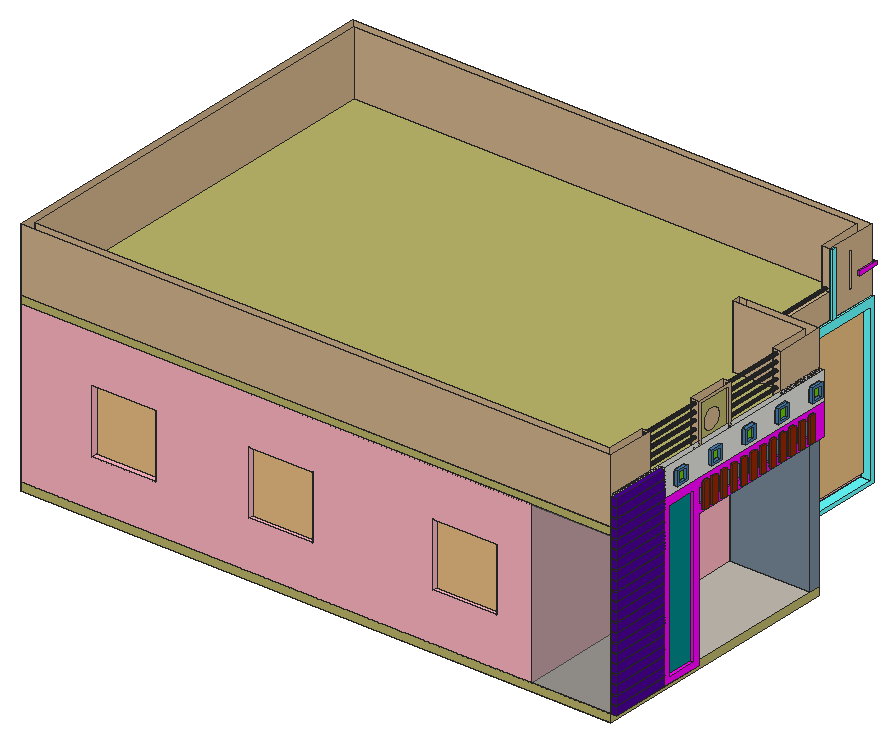
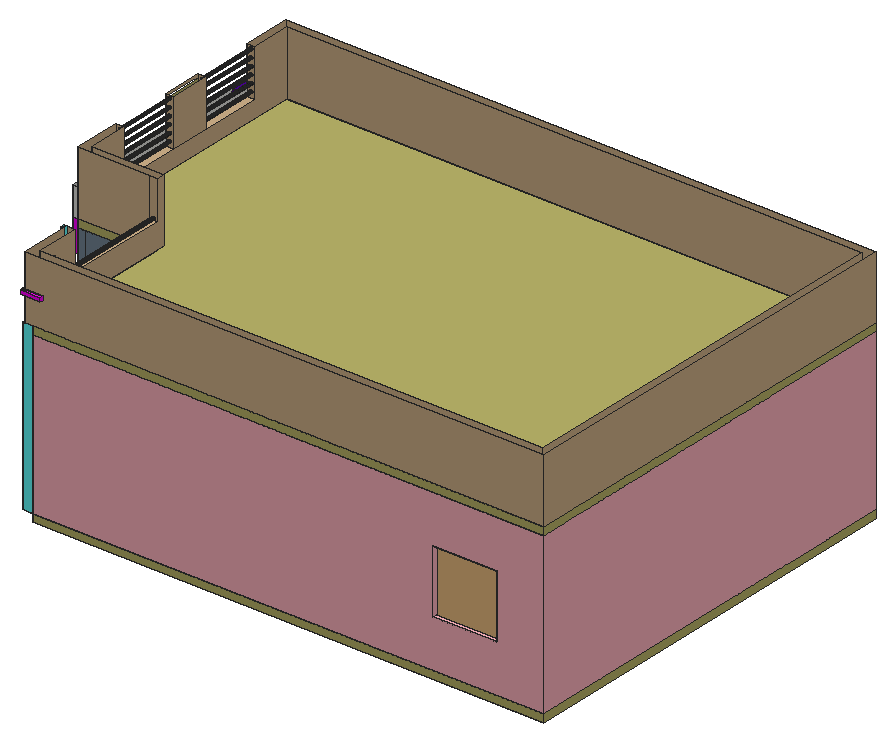
# SketchUp Ruby script. Lengths in inches.
U = 1.inch
M = Sketchup.active_model
def pt(a) = Geom::Point3d.new(a.map { |v| v * U })
def face(e, loops, mat)
  f = e.add_face(loops[0].map { |a| pt(a) })
  loops[1..].each { |l| e.add_face(l.map { |a| pt(a) }).erase! }
  f.material = f.back_material = mat if mat
  f
end
# faces: each face lists its corners as indices into pts; further lists are holes
def faces(e, pts, list, mat = nil) = list.each { |f| face(e, (f[0].is_a?(Array) ? f : [f]).map { |l| l.map { |i| pts[i] } }, mat) }
# xy, xz, yz: faces in a plane at the given z, y or x. An outline is a flat list of corners, or four numbers for a rectangle; further outlines are holes
def ring(l) = l.size == 4 ? [[l[0], l[1]], [l[2], l[1]], [l[2], l[3]], [l[0], l[3]]] : l.each_slice(2).to_a
def flat(e, list, mat, &to3) = list.each { |f| face(e, (f[0].is_a?(Array) ? f : [f]).map { |l| ring(l).map { |u, v| to3.(u, v) } }, mat) }
def xy(e, z, list, mat = nil) = flat(e, list, mat) { |x, y| [x, y, z] }
def xz(e, y, list, mat = nil) = flat(e, list, mat) { |x, z| [x, y, z] }
def yz(e, x, list, mat = nil) = flat(e, list, mat) { |y, z| [x, y, z] }
def lines(e, pts, list) = list.each { |a, b| e.add_line(pt(pts[a]), pt(pts[b])) }
# prism: a flat outline (further loops are holes) pulled along v
def prism(e, loops, v, mat = nil)
  f = face(e, loops, mat); d = Geom::Vector3d.new(v.map { |x| x * U })
  f.pushpull(f.normal.samedirection?(d) ? d.length : -d.length)
end
def box(e, o, s, mat = nil) = prism(e, [[o, [o[0] + s[0], o[1], o[2]], [o[0] + s[0], o[1] + s[1], o[2]], [o[0], o[1] + s[1], o[2]]]], [0, 0, s[2]], mat)
def at(x, y, z, deg = 0) = Geom::Transformation.translation(pt([x, y, z])) * Geom::Transformation.rotation(ORIGIN, Z_AXIS, deg.degrees)
def axes(o, x, y, z) = Geom::Transformation.new([*x, 0, *y, 0, *z, 0, *pt(o).to_a, 1])
def part(name) = M.definitions.add(name)
# library, detail: a bought-in or finely detailed component or shape, given as its bounding box
def library(name, o, s) = part(name).tap { |d| box(d.entities, o, s) }
def detail(e, o, s) = box(e.add_group.entities, o, s)
def put(e, d, t, mat = nil) = e.add_instance(d, t).tap { |i| i.material = mat if mat }
def group(e, t, mat = nil) = e.add_group.tap { |g| g.transformation = t; g.material = mat if mat }.entities
root = M.entities
M.materials.add("[0003_DeepPink]").color = [255, 20, 147]
M.materials.add("[0005_LightPink]").color = [255, 182, 193]
M.materials.add("[0035_Tan]").color = [210, 180, 140]
M.materials.add("[0057_DarkKhaki]").color = [189, 183, 107]
M.materials.add("[0080_DarkCyan]").color = [0, 139, 139]
M.materials.add("[0100_SteelBlue]").color = [70, 130, 180]
M.materials.add("[0109_DarkSlateBlue]").color = [72, 61, 139]
M.materials.add("[0110_LightSlateGray]").color = [119, 136, 153]
M.materials.add("[0127_Magenta]").color = [255, 0, 255]
M.materials.add("[0136_Charcoal]").color = [35, 35, 35]
M.materials.add("[Color B07]").color = [153, 38, 0]
M.materials.add("[Color F06]").color = [102, 204, 0]
M.materials.add("[Color H03]").color = [101, 255, 255]
M.materials.add("[Color J07]").color = [76, 0, 153]
M.materials.add("[Field Rectangle Tile]").color = [196, 189, 179]
M.materials.add("[Translucent Glass Gray]").color = [128, 128, 128]
M.materials["[Translucent Glass Gray]"].alpha = 0.5
c1 = library("BED 3",[-244.73,-59.6875,196.6875],[91.01,69.4,39.64])
c2 = library("建立群組\#166",[-1.39,17.71,0],[5.33,43.31,86.61])
c3 = library("Группа\#16",[0,0,0],[5.38,37.87,81.85])
c4 = library("Component",[269.12,209.03,0],[24,4.72,84.37])
c5 = library("Group\#20",[0,0,6],[2,110.9,114])
c6 = library("mesh-166",[-1553.69,-2604.3125,-42.18],[1702.88,1401.6,88.28])
c7 = part("Group17")
put(c7.entities,c6,at(294.66,859.51,3.5))
c8 = library("mesh-158",[272.88,-1887.9,-41.96],[1017.57,1401.85,65.81])
c9 = part("Component\#4")
box(c9.entities,[2.75,0,0],[18.9375,4.3125,2],"[Color B07]")
c10 = part("Component\#3")
xy(c10.entities,0,[[0,0,3,9.4375]],"[0100_SteelBlue]")
xy(c10.entities,1.08,[[0,1.08,0.1875,8.36],[0.1875,1.08,3,8.36]],"[0100_SteelBlue]")
xy(c10.entities,9.29,[[0,1.08,0.1875,8.36],[0.1875,1.08,3,8.36]],"[0100_SteelBlue]")
xy(c10.entities,10.375,[[0,0,3,9.4375]],"[0100_SteelBlue]")
xz(c10.entities,0,[[0,0,3,10.375]],"[0100_SteelBlue]")
xz(c10.entities,1.08,[[0,1.08,0.1875,9.29],[0.1875,1.08,3,9.29]],"[0100_SteelBlue]")
xz(c10.entities,8.36,[[0,1.08,0.1875,9.29],[0.1875,1.08,3,9.29]],"[0100_SteelBlue]")
xz(c10.entities,9.4375,[[0,0,3,10.375]],"[0100_SteelBlue]")
yz(c10.entities,0,[[[0,0,9.4375,10.375],[1.08,1.08,8.36,9.29]]],"[0100_SteelBlue]")
yz(c10.entities,0.1875,[[1.08,1.08,8.36,9.29]],"[Color F06]")
yz(c10.entities,3,[[[0,0,9.4375,10.375],[1.08,1.08,8.36,9.29]]],"[0100_SteelBlue]")
c11 = part("Round post")
xy(c11.entities,0,[[1,0,0.74,0.03,0.5,0.13,0.29,0.29,0.13,0.5,0.03,0.74,0,1,0.03,1.26,0.13,1.5,0.29,1.71,0.5,1.87,0.74,1.97,1,2,1.26,1.97,1.5,1.87,1.71,1.71,1.87,1.5,1.97,1.26,2,1,1.97,0.74,1.87,0.5,1.71,0.29,1.5,0.13,1.26,0.03]],"[0035_Tan]")
xy(c11.entities,46.55,[[1,0,1.26,0.03,1.5,0.13,1.71,0.29,1.87,0.5,1.97,0.74,2,1,1.97,1.26,1.87,1.5,1.71,1.71,1.5,1.87,1.26,1.97,1,2,0.74,1.97,0.5,1.87,0.29,1.71,0.13,1.5,0.03,1.26,0,1,0.03,0.74,0.13,0.5,0.29,0.29,0.5,0.13,0.74,0.03]],"[0035_Tan]")
p = [[0.5,0.13,0],[0.74,0.03,0],[0.74,0.03,46.55],[0.5,0.13,46.55],[1,0,0],[1,0,46.55],
  [1.26,0.03,0],[1.26,0.03,46.55],[1.5,0.13,0],[1.5,0.13,46.55],[0.29,0.29,0],[0.29,0.29,46.55],
  [1.71,0.29,0],[1.71,0.29,46.55],[0.13,0.5,0],[0.13,0.5,46.55],[1.87,0.5,0],[1.87,0.5,46.55],
  [0.03,0.74,0],[0.03,0.74,46.55],[1.97,0.74,0],[1.97,0.74,46.55],[0,1,0],[0,1,46.55],
  [2,1,0],[2,1,46.55],[0.03,1.26,0],[0.03,1.26,46.55],[1.97,1.26,0],[1.97,1.26,46.55],
  [0.13,1.5,0],[0.13,1.5,46.55],[1.87,1.5,0],[1.87,1.5,46.55],[0.29,1.71,0],[0.29,1.71,46.55],
  [1.71,1.71,0],[1.71,1.71,46.55],[0.5,1.87,0],[0.5,1.87,46.55],[1.5,1.87,0],[1.5,1.87,46.55],
  [0.74,1.97,0],[0.74,1.97,46.55],[1.26,1.97,0],[1.26,1.97,46.55],[1,2,0],[1,2,46.55]]
faces(c11.entities,p,[[0,1,2,3],[1,4,5,2],[4,6,7,5],[6,8,9,7],[10,0,3,11],[8,12,13,9],[14,10,11,15],[12,16,17,13],
  [18,14,15,19],[16,20,21,17],[22,18,19,23],[20,24,25,21],[26,22,23,27],[24,28,29,25],[30,26,27,31],[28,32,33,29],
  [34,30,31,35],[32,36,37,33],[38,34,35,39],[36,40,41,37],[42,38,39,43],[40,44,45,41],[46,42,43,47],[44,46,47,45]],"[0136_Charcoal]")
c12 = part("Group\#26")
put(c12.entities,c11,axes([2,11.53,0],[-1,0,0],[0,1,0],[0,0,-1]))
put(c12.entities,c11,axes([2,17.29,0],[-1,0,0],[0,1,0],[0,0,-1]))
put(c12.entities,c11,axes([2,5.76,0],[-1,0,0],[0,1,0],[0,0,-1]))
put(c12.entities,c11,axes([2,23.05,0],[-1,0,0],[0,1,0],[0,0,-1]))
put(c12.entities,c11,axes([2,28.8125,0],[-1,0,0],[0,1,0],[0,0,-1]))
put(c12.entities,c11,axes([2,0,0],[-1,0,0],[0,1,0],[0,0,-1]))
c13 = part("Group\#24")
prism(c13.entities,[[[2.25,1.125,0],[2.21,0.83,0],[2.1,0.5625,0],[1.92,0.33,0],[1.6875,0.15,0],[1.42,0.04,0],[1.125,0,0],[0.83,0.04,0],[0.5625,0.15,0],[0.33,0.33,0],[0.15,0.5625,0],[0.04,0.83,0],[0,1.125,0],[0.04,1.42,0],[0.15,1.6875,0],[0.33,1.92,0],[0.5625,2.1,0],[0.83,2.21,0],[1.125,2.25,0],[1.42,2.21,0],[1.6875,2.1,0],[1.92,1.92,0],[2.1,1.6875,0],[2.21,1.42,0]]],[0,0,77.9])
c14 = part("Component\#2")
xy(c14.entities,-13,[[13.51,0,15.51,2.94]],"[0127_Magenta]")
xy(c14.entities,2,[[0,0,15.51,2.94]],"[0127_Magenta]")
xz(c14.entities,0,[[13.51,-13,15.51,0],[0,0,15.51,2]],"[0127_Magenta]")
xz(c14.entities,2.94,[[13.51,-13,15.51,2],[0,0,13.51,2]],"[0127_Magenta]")
yz(c14.entities,0,[[0,0,2.94,2]],"[0127_Magenta]")
yz(c14.entities,13.51,[[0,-13,2.94,2]],"[0127_Magenta]")
yz(c14.entities,15.51,[[0,-13,2.94,2]],"[0127_Magenta]")
xy(root,0,[[384,188.1,444,197.1]],"[0109_DarkSlateBlue]")
xy(root,0,[[444,2,448,79.01]],"[Color J07]")
xy(root,4,[[445,51.2,448,75.01]],"[0127_Magenta]")
xy(root,6,[[444,2,448,47.2]],"[Color J07]")
xy(root,7,[[444,2,448,47.2]])
xy(root,13,[[444,2,448,47.2]],"[Color J07]")
xy(root,14,[[444,2,448,47.2]])
xy(root,20,[[444,2,448,47.2]],"[Color J07]")
xy(root,21,[[444,2,448,47.2]])
xy(root,27,[[444,2,448,47.2]],"[Color J07]")
xy(root,28,[[444,2,448,47.2]])
xy(root,34,[[444,2,448,47.2]],"[Color J07]")
xy(root,35,[[444,2,448,47.2]],"[Color J07]")
xy(root,41,[[444,2,448,47.2]],"[Color J07]")
xy(root,42,[[444,2,448,47.2]],"[Color J07]")
xy(root,48,[[444,2,448,47.2]],"[Color J07]")
xy(root,49,[[444,2,448,47.2]],"[Color J07]")
xy(root,55,[[444,2,448,47.2]],"[Color J07]")
xy(root,56,[[444,2,448,47.2]],"[Color J07]")
xy(root,62,[[444,2,448,47.2]],"[Color J07]")
xy(root,63,[[444,2,448,47.2]],"[Color J07]")
xy(root,69,[[444,2,448,47.2]],"[Color J07]")
xy(root,70,[[444,2,448,47.2]],"[Color J07]")
xy(root,76,[[444,2,448,47.2]],"[Color J07]")
xy(root,77,[[444,2,448,47.2]],"[Color J07]")
xy(root,83,[[444,2,448,47.2]],"[Color J07]")
xy(root,84,[[444,2,448,47.2]],"[Color J07]")
xy(root,90,[[444,2,448,47.2]],"[Color J07]")
xy(root,91,[[444,2,448,47.2]],"[Color J07]")
xy(root,97,[[444,2,448,47.2]],"[Color J07]")
xy(root,98,[[444,2,448,47.2]],"[Color J07]")
xy(root,102,[[444,79.01,448,197.1]],"[0127_Magenta]")
xy(root,104,[[444,2,448,47.2]],"[Color J07]")
xy(root,105,[[444,2,448,47.2]],"[Color J07]")
xy(root,108,[[444,79.01,446,188.1],[446,79.01,448,188.1]],"[0127_Magenta]")
xy(root,111,[[444,2,448,47.2]],"[Color J07]")
xy(root,112,[[444,2,448,47.2]],"[Color J07]")
xy(root,118,[[444,2,448,47.2]],"[Color J07]")
xy(root,119,[[444,2,448,47.2]],"[Color J07]")
xy(root,119.875,[[445,51.2,448,75.01],[444,79.01,446,188.1],[446,79.01,448,188.1]],"[0127_Magenta]")
xy(root,120,[[384,188.1,444,197.1]],"[0109_DarkSlateBlue]")
xy(root,125,[[444,2,448,47.2]],"[Color J07]")
xy(root,126,[[[0,2,0,314,390,314,390,197.1,444,197.1,444,2],[6,8,438,8,438,191.1,384,191.1,384,308,6,308]]],"[0035_Tan]")
xy(root,126,[[444,2,448,47.2]],"[Color J07]")
xy(root,132,[[444,2,448,47.2]],"[Color J07]")
xy(root,133,[[444,2,448,47.2]],"[Color J07]")
xy(root,138.27,[[384,292.3,390,295.12]],"[0035_Tan]")
xy(root,138.5,[[438,38,444,84.55],[438,84.55,444,114.55],[438,114.55,444,161.1]],"[0035_Tan]")
xy(root,139,[[444,2,448,47.2]],"[Color J07]")
xy(root,140,[[444,2,448,47.2]],"[Color J07]")
xy(root,140.5,[[442,86.55,444,112.55]],"[0035_Tan]")
xy(root,145.18,[[384,197.1,390,275]],"[0035_Tan]")
xy(root,146,[[444,2,448,47.2]],"[Color J07]")
xz(root,2,[[0,126,444,174]],"[0035_Tan]")
xz(root,2,[[444,0,448,6],[444,7,448,13],[444,14,448,20],[444,21,448,27],[444,28,448,34],
  [444,35,448,41],[444,42,448,48],[444,49,448,55],[444,56,448,62],[444,63,448,69],
  [444,70,448,76],[444,77,448,83],[444,84,448,90],[444,91,448,97],[444,98,448,104],
  [444,105,448,111],[444,112,448,118],[444,119,448,125],[444,126,448,132],[444,133,448,139],
  [444,140,448,146]],"[Color J07]")
xz(root,2,[[384,0,444,120]],"[Translucent Glass Gray]")
xz(root,8,[[6,126,438,174]],"[0035_Tan]")
xz(root,38,[[438,138.5,444,174]],"[0035_Tan]")
xz(root,47.2,[[444,6,448,7],[444,13,448,14],[444,20,448,21],[444,27,448,28],[444,34,448,35],
  [444,41,448,42],[444,48,448,49],[444,55,448,56],[444,62,448,63],[444,69,448,70],
  [444,76,448,77],[444,83,448,84],[444,90,448,91],[444,97,448,98],[444,104,448,105],
  [444,111,448,112],[444,118,448,119],[444,125,448,126],[444,132,448,133],[444,139,448,140],
  [444,146,448,147]])
xz(root,51.2,[[445,4,448,119.875]],"[0127_Magenta]")
xz(root,75.01,[[445,4,448,119.875]],"[0127_Magenta]")
xz(root,79.01,[[444,0,448,102],[444,102,448,108],[444,108,446,119.875],[446,108,448,119.875]],"[0127_Magenta]")
xz(root,84.55,[[438,138.5,444,174]],"[0035_Tan]")
xz(root,86.55,[[442,140.5,444,172]],"[0035_Tan]")
xz(root,112.55,[[442,140.5,444,172]],"[0035_Tan]")
xz(root,114.55,[[438,138.5,444,174]],"[0035_Tan]")
xz(root,161.1,[[438,138.5,444,174]],"[0035_Tan]")
xz(root,188.1,[[384,0,444,120]],"[0110_LightSlateGray]")
xz(root,188.1,[[446,108,448,119.875]],"[0127_Magenta]")
xz(root,191.1,[[384,126,438,174]],"[0035_Tan]")
xz(root,197.1,[[444,126,448,147.28]])
xz(root,197.1,[[390,126,444,174],[384,145.18,390,174]],"[0035_Tan]")
xz(root,197.1,[[384,0,438,120],[438,0,444,120]],"[0110_LightSlateGray]")
xz(root,197.1,[[444,102,448,126]],"[0127_Magenta]")
xz(root,275,[[384,145.18,390,174]],"[0035_Tan]")
xz(root,292.3,[[384,138.27,390,165.21]],"[0035_Tan]")
xz(root,295.12,[[384,138.27,390,165.21]],"[0035_Tan]")
xz(root,308,[[6,126,384,174]],"[0035_Tan]")
xz(root,314,[[0,126,390,174]],"[0035_Tan]")
yz(root,0,[[2,126,314,174]],"[0035_Tan]")
yz(root,6,[[8,126,308,174]],"[0035_Tan]")
yz(root,384,[[[191.1,126,191.1,174,197.1,174,197.1,145.18,275,145.18,275,174,308,174,308,126],[292.3,138.27,295.12,165.21]]],"[0035_Tan]")
yz(root,384,[[188.1,0,197.1,120]],"[0109_DarkSlateBlue]")
yz(root,390,[[197.1,126,275,145.18],[[278,126,314,174],[292.3,138.27,295.12,165.21]]],"[0035_Tan]")
yz(root,438,[[8,126,8,174,38,174,38,138.5,161.1,138.5,161.1,174,191.1,174,191.1,126],[84.55,138.5,114.55,174]],"[0035_Tan]")
yz(root,442,[[[86.55,140.5,112.55,172],[98.5,147.98,98.02,148.01,97.54,148.07,97.0625,148.16,96.59,148.28,96.13,148.43,95.69,148.61,95.25,148.82,94.82,149.05,94.42,149.3125,94.03,149.6,93.65,149.91,93.3,150.24,92.97,150.59,92.66,150.96,92.38,151.35,92.12,151.76,91.89,152.1875,91.68,152.625,91.51,153.07,91.36,153.53,91.24,154,91.15,154.48,91.09,154.96,91.06,155.4375,91.06,155.92,91.09,156.41,91.15,156.88,91.24,157.36,91.36,157.83,91.51,158.29,91.69,158.74,91.9,159.17,92.13,159.6,92.39,160.01,92.67,160.4,92.98,160.77,93.3125,161.12,93.67,161.45,94.04,161.76,94.43,162.04,94.84,162.3,95.26,162.53,95.7,162.74,96.15,162.92,96.61,163.07,97.08,163.1875,97.55,163.28,98.03,163.34,98.52,163.37,99,163.37,99.48,163.33,99.96,163.27,100.4375,163.18,100.9,163.0625,101.36,162.91,101.8125,162.73,102.25,162.53,102.67,162.29,103.08,162.03,103.47,161.75,103.85,161.44,104.2,161.11,104.53,160.76,104.84,160.38,105.12,159.99,105.38,159.58,105.61,159.16,105.82,158.72,105.99,158.27,106.14,157.8125,106.26,157.34,106.35,156.87,106.41,156.39,106.44,155.91,106.44,155.42,106.41,154.94,106.35,154.46,106.26,153.99,106.14,153.52,105.99,153.06,105.81,152.61,105.6,152.17,105.37,151.75,105.11,151.34,104.83,150.95,104.52,150.58,104.1875,150.22,103.83,149.89,103.46,149.59,103.07,149.3,102.66,149.04,102.24,148.8125,101.8,148.61,101.35,148.43,100.89,148.28,100.42,148.16,99.95,148.07,99.47,148.01,98.98,147.98]]],"[0057_DarkKhaki]")
yz(root,444,[[2,0,2,6,47.2,6,47.2,7,2,7,2,13,47.2,13,47.2,14,2,14,2,20,47.2,20,47.2,21,2,21,2,27,47.2,27,47.2,28,2,28,2,34,47.2,34,47.2,35,2,35,2,41,47.2,41,47.2,42,2,42,2,48,47.2,48,47.2,49,2,49,2,55,47.2,55,47.2,56,2,56,2,62,47.2,62,47.2,63,2,63,2,69,47.2,69,47.2,70,2,70,2,76,47.2,76,47.2,77,2,77,2,83,47.2,83,47.2,84,2,84,2,90,47.2,90,47.2,91,2,91,2,97,47.2,97,47.2,98,2,98,2,104,47.2,104,47.2,105,2,105,2,111,47.2,111,47.2,112,2,112,2,118,47.2,118,47.2,119,2,119,2,125,47.2,125,47.2,126,2,126,2,132,47.2,132,47.2,133,2,133,2,139,47.2,139,47.2,140,2,140,2,146,47.2,146,47.2,147,2,147,2,147.28,197.1,147.28,197.1,120,188.1,120,188.1,119.875,79.01,119.875,79.01,0],[2,6,47.2,7],[2,13,47.2,14],[2,20,47.2,21],[2,27,47.2,28],
  [2,34,47.2,35],[2,41,47.2,42],[2,48,47.2,49],[2,55,47.2,56],[2,62,47.2,63],
  [2,69,47.2,70],[2,76,47.2,77],[2,83,47.2,84],[2,97,47.2,98],[2,104,47.2,105],
  [2,111,47.2,112],[2,118,47.2,119]])
yz(root,444,[[2,126,38,174],[38,126,161.1,138.5],[161.1,126,197.1,174],[[84.55,138.5,114.55,174],[86.55,140.5,112.55,172]]],"[0035_Tan]")
yz(root,444,[[188.1,102,197.1,120]],"[0109_DarkSlateBlue]")
yz(root,444,[[188.1,0,197.1,102]],"[0110_LightSlateGray]")
yz(root,444,[[79.01,102,188.1,108],[79.01,108,188.1,119.875]],"[0127_Magenta]")
yz(root,444,[[2,90,47.2,91]],"[Color J07]")
yz(root,445,[[51.2,4,75.01,119.875]],"[0080_DarkCyan]")
yz(root,446,[[79.01,108,188.1,119.875]],"[0110_LightSlateGray]")
yz(root,448,[[[47.2,0,79.01,0,79.01,102,197.1,102,197.1,126,47.2,126],[51.2,4,75.01,119.875],[79.01,108,188.1,119.875]]],"[0127_Magenta]")
yz(root,448,[[2,0,47.2,6],[2,7,47.2,13],[2,14,47.2,20],[2,21,47.2,27],[2,28,47.2,34],
  [2,35,47.2,41],[2,42,47.2,48],[2,49,47.2,55],[2,56,47.2,62],[2,63,47.2,69],
  [2,70,47.2,76],[2,77,47.2,83],[2,84,47.2,90],[2,91,47.2,97],[2,98,47.2,104],
  [2,105,47.2,111],[2,112,47.2,118],[2,119,47.2,125],[2,126,47.2,132],[2,133,47.2,139],
  [2,140,47.2,146]],"[Color J07]")
g1 = group(root,at(0,2,-6))
xy(g1,0,[[0,0,0,312,384,312,384,195.1,444,195.1,444,0]],"[0057_DarkKhaki]")
xy(g1,6,[[0,0,444,0,444,195.1,384,195.1,384,312,0,312]],"[Field Rectangle Tile]")
xz(g1,0,[[0,0,444,6]],"[0057_DarkKhaki]")
xz(g1,195.1,[[384,0,444,6]],"[0057_DarkKhaki]")
xz(g1,312,[[0,0,384,6]],"[0057_DarkKhaki]")
yz(g1,0,[[0,0,312,6]],"[0057_DarkKhaki]")
yz(g1,384,[[195.1,0,312,6]],"[0057_DarkKhaki]")
yz(g1,444,[[0,0,195.1,6]],"[0057_DarkKhaki]")
g2 = group(root,at(384,197.1,-6),"[Color H03]")
prism(g2,[[[8,0,6],[8,116.9,6],[8,116.9,132],[8,0,132]],[[8,3,126],[8,113.9,126],[8,113.9,9],[8,3,9]]],[-8,0,0])
p = [[0,116.9,6],[0,116.9,0]]
lines(g2,p,[[0,1]])
put(root,c1,axes([250.03,214.22,-197.57],[1,0,0],[0,-1,0],[0,0,1]))
put(root,c1,at(250.03,106.31,-197.57))
put(root,c2,axes([292.96,170.63,84],[0,0.81344,0],[-0.69372,0,0],[0,0,-0.96982]))
put(root,c3,axes([381.06,158.9,0],[-0.99999,-0.00519,0],[0.00503,-0.96999,0],[0,0,1.02626]))
put(root,c2,axes([145.5,217.51,84],[-0.81344,0,0],[0,-0.69372,0],[0,0,-0.96982]))
g3 = group(root,at(0,2,0))
xy(g3,0,[[0,0,0,312,384,312,384,156.17,375,156.17,375,303,9,303,9,9,375,9,375,120.17,384,120.17,384,0],[288.5,9,288.5,119.5,298.1,119.5,298.1,115,293,115,293,9],[328.1,115,375,119.5],[239.5,167.5,239.5,303,244,303,244,172,250.625,172,250.625,167.5],[280.625,167.5,375,172]],"[0005_LightPink]")
xy(g3,36,[[53.66,0,101.66,9],[171.87,0,219.87,9],[309.9,0,357.9,9],[375,77.01,384,101.01],[375,202.66,384,250.66],
  [35.36,303,83.36,312]],"[0005_LightPink]")
xy(g3,72,[[375,77.01,384,101.01]],"[0005_LightPink]")
xy(g3,84,[[53.66,0,101.66,9],[171.87,0,219.87,9],[309.9,0,357.9,9],[298.1,115,328.1,119.5],[375,120.17,384,156.17],
  [141,132.29,145.5,162.29],[250.625,167.5,280.625,172],[141,173.18,145.5,203.18],[375,202.66,384,250.66],[150.23,246,174.23,250.5],
  [35.36,303,83.36,312]],"[0005_LightPink]")
xy(g3,120,[[[0,0,384,312],[9,9,375,303]],[141,9,145.5,9,145.5,303,141,303,141,169.5,9,169.5,9,165,141,165],[288.5,9,293,9,293,115,375,115,375,119.5,288.5,119.5],[239.5,167.5,375,167.5,375,172,244,172,244,303,239.5,303],[145.5,246,239.5,250.5]],"[0005_LightPink]")
xz(g3,0,[[[0,0,384,120],[309.9,36,357.9,84],[171.87,36,219.87,84],[53.66,36,101.66,84]]],"[0005_LightPink]")
xz(g3,9,[[[9,0,141,120],[53.66,36,101.66,84]],[[145.5,0,288.5,120],[171.87,36,219.87,84]],[288.5,0,293,120],[[293,0,375,120],[309.9,36,357.9,84]]],"[0005_LightPink]")
xz(g3,77.01,[[375,36,384,72]],"[0005_LightPink]")
xz(g3,101.01,[[375,36,384,72]],"[0005_LightPink]")
xz(g3,115,[[293,0,298.1,0,298.1,84,328.1,84,328.1,0,375,0,375,120,293,120]],"[0005_LightPink]")
xz(g3,119.5,[[288.5,0,288.5,120,375,120,375,0,328.1,0,328.1,84,298.1,84,298.1,0]],"[0005_LightPink]")
xz(g3,120.17,[[375,0,384,84]],"[0005_LightPink]")
xz(g3,132.29,[[141,0,145.5,84]],"[0005_LightPink]")
xz(g3,156.17,[[375,0,384,84]],"[0005_LightPink]")
xz(g3,162.29,[[141,0,145.5,84]],"[0005_LightPink]")
xz(g3,165,[[9,0,141,120]],"[0005_LightPink]")
xz(g3,167.5,[[239.5,0,250.625,0,250.625,84,280.625,84,280.625,0,375,0,375,120,239.5,120]],"[0005_LightPink]")
xz(g3,169.5,[[9,0,141,120]],"[0005_LightPink]")
xz(g3,172,[[244,0,244,120,375,120,375,0,280.625,0,280.625,84,250.625,84,250.625,0]],"[0005_LightPink]")
xz(g3,173.18,[[141,0,145.5,84]],"[0005_LightPink]")
xz(g3,202.66,[[375,36,384,84]],"[0005_LightPink]")
xz(g3,203.18,[[141,0,145.5,84]],"[0005_LightPink]")
xz(g3,246,[[145.5,0,150.23,0,150.23,84,174.23,84,174.23,0,239.5,0,239.5,120,145.5,120]],"[0005_LightPink]")
xz(g3,250.5,[[145.5,0,145.5,120,239.5,120,239.5,0,174.23,0,174.23,84,150.23,84,150.23,0]],"[0005_LightPink]")
xz(g3,250.66,[[375,36,384,84]],"[0005_LightPink]")
xz(g3,303,[[[9,0,141,120],[35.36,36,83.36,84]],[145.5,0,239.5,120],[239.5,0,244,120],[244,0,375,120]],"[0005_LightPink]")
xz(g3,312,[[[0,0,384,120],[35.36,36,83.36,84]]],"[0005_LightPink]")
yz(g3,0,[[0,0,312,120]],"[0005_LightPink]")
yz(g3,9,[[9,0,165,120],[169.5,0,303,120]],"[0005_LightPink]")
yz(g3,35.36,[[303,36,312,84]],"[0005_LightPink]")
yz(g3,53.66,[[0,36,9,84]],"[0005_LightPink]")
yz(g3,83.36,[[303,36,312,84]],"[0005_LightPink]")
yz(g3,101.66,[[0,36,9,84]],"[0005_LightPink]")
yz(g3,141,[[9,0,9,120,165,120,165,0,162.29,0,162.29,84,132.29,84,132.29,0],[169.5,0,169.5,120,303,120,303,0,203.18,0,203.18,84,173.18,84,173.18,0]],"[0005_LightPink]")
yz(g3,145.5,[[9,0,132.29,0,132.29,84,162.29,84,162.29,0,173.18,0,173.18,84,203.18,84,203.18,0,246,0,246,120,9,120],[250.5,0,303,120]],"[0005_LightPink]")
yz(g3,150.23,[[246,0,250.5,84]],"[0005_LightPink]")
yz(g3,171.87,[[0,36,9,84]],"[0005_LightPink]")
yz(g3,174.23,[[246,0,250.5,84]],"[0005_LightPink]")
yz(g3,219.87,[[0,36,9,84]],"[0005_LightPink]")
yz(g3,239.5,[[167.5,0,246,120],[246,0,250.5,120],[250.5,0,303,120]],"[0005_LightPink]")
yz(g3,244,[[172,0,303,120]],"[0005_LightPink]")
yz(g3,250.625,[[167.5,0,172,84]],"[0005_LightPink]")
yz(g3,280.625,[[167.5,0,172,84]],"[0005_LightPink]")
yz(g3,288.5,[[9,0,119.5,120]],"[0005_LightPink]")
yz(g3,293,[[9,0,115,120]],"[0005_LightPink]")
yz(g3,298.1,[[115,0,119.5,84]],"[0005_LightPink]")
yz(g3,309.9,[[0,36,9,84]],"[0005_LightPink]")
yz(g3,328.1,[[115,0,119.5,84]],"[0005_LightPink]")
yz(g3,357.9,[[0,36,9,84]],"[0005_LightPink]")
yz(g3,375,[[[9,0,115,120],[77.01,36,101.01,72]],[115,0,119.5,120],[119.5,0,119.5,120,167.5,120,167.5,0,156.17,0,156.17,84,120.17,84,120.17,0],[167.5,0,172,120],[[172,0,303,120],[202.66,36,250.66,84]]],"[0005_LightPink]")
yz(g3,384,[[[0,0,120.17,0,120.17,84,156.17,84,156.17,0,198.1,0,198.1,120,0,120],[77.01,36,101.01,72]],[[198.1,0,312,120],[202.66,36,250.66,84]]],"[0005_LightPink]")
p = [[384,156.17,0],[384,120.17,0]]
lines(g3,p,[[0,1]])
put(root,c4,at(-118.89,38.97,0))
put(root,c2,axes([145.5,176.62,84],[-0.81344,0,0],[0,-0.69372,0],[0,0,-0.96982]))
put(root,c5,at(384,200.1,0),"[0003_DeepPink]")
put(root,c7,axes([322.41,6.55,95.75],[-0.02819,0,0],[0,0,0.03425],[0,0.02402,0]))
put(root,c7,axes([66.17,7.43,95.75],[-0.02819,0,0],[0,0,0.03425],[0,0.02402,0]))
put(root,c7,axes([184.375,6.55,95.75],[-0.02819,0,0],[0,0,0.03425],[0,0.02402,0]))
put(root,c7,axes([47.87,309.75,95.75],[-0.02819,0,0],[0,0,0.03425],[0,0.02402,0]))
g4 = group(root,at(378.71,90.96,54))
put(g4,c8,axes([0.38,-18.39,30.49],[0,0.02359,0],[0,0,0.02568],[-0.03937,0,0]))
put(root,c7,axes([379.64,240.15,95.75],[0,0.02819,0],[0,0,0.03425],[0.02402,0,0]))
put(root,c9,axes([448,90.02,126],[0,0,-1],[0,1,0],[1,0,0]))
put(root,c9,axes([448,99.17,126],[0,0,-1],[0,1,0],[1,0,0]))
put(root,c9,axes([448,108.33,126],[0,0,-1],[0,1,0],[1,0,0]))
put(root,c9,axes([448,117.49,126],[0,0,-1],[0,1,0],[1,0,0]))
put(root,c9,axes([448,126.64,126],[0,0,-1],[0,1,0],[1,0,0]))
put(root,c9,axes([448,135.8,126],[0,0,-1],[0,1,0],[1,0,0]))
put(root,c9,axes([448,144.95,126],[0,0,-1],[0,1,0],[1,0,0]))
put(root,c9,axes([448,154.11,126],[0,0,-1],[0,1,0],[1,0,0]))
put(root,c9,axes([448,163.27,126],[0,0,-1],[0,1,0],[1,0,0]))
put(root,c9,axes([448,172.42,126],[0,0,-1],[0,1,0],[1,0,0]))
put(root,c9,axes([448,181.58,126],[0,0,-1],[0,1,0],[1,0,0]))
put(root,c9,axes([448,82.14,126],[0,0,-1],[0,1,0],[1,0,0]))
g5 = group(root,at(0,2,120),"[Color J07]")
prism(g5,[[[0,312,0],[384,312,0],[384,195.1,0],[444,195.1,0],[444,0,0],[0,0,0]]],[0,0,6],"[0057_DarkKhaki]")
g6 = group(root,at(390,275,126),"[Color H03]")
box(g6,[0,0,0],[2,3,48])
g7 = group(root,at(448,47.2,126))
yz(g7,0,[[0,0,149.9,21.28]])
put(root,c10,at(448,55.85,131.77))
put(root,c10,at(448,87.57,131.77))
put(root,c10,at(448,119.28,131.77))
put(root,c10,at(448,151,131.77))
put(root,c10,at(448,182.72,131.77))
put(root,c12,axes([439.77,38,141.77],[1,0,0],[0,0,1],[0,-1,0]))
put(root,c12,axes([439.77,114.55,141.77],[1,0,0],[0,0,1],[0,-1,0]))
put(root,c13,axes([385.75,275,145.18],[1,0,0],[0,0,1],[0,-1,0]),"[0136_Charcoal]")
put(root,c14,axes([390,300.49,145.72],[0,1,0],[0,0,1],[1,0,0]))
